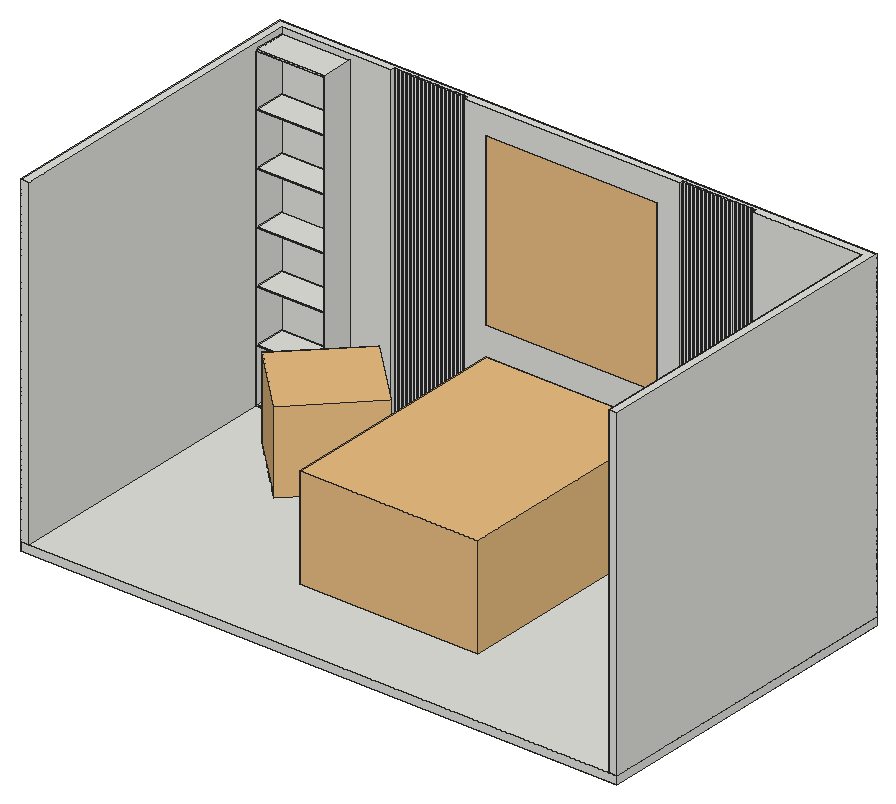
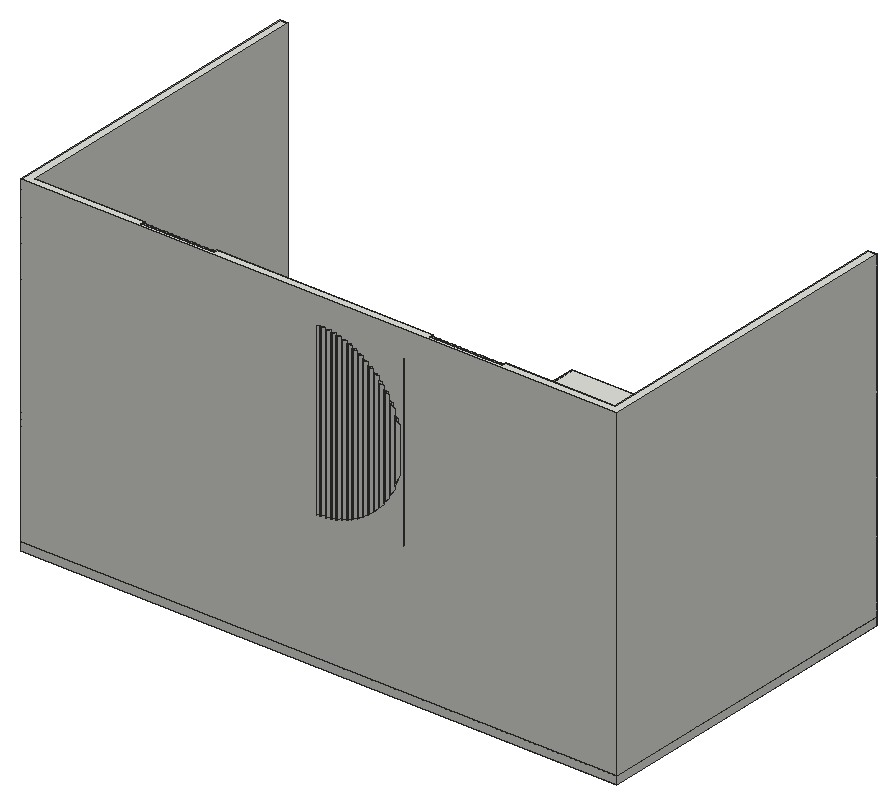
# SketchUp Ruby script. Lengths in inches.
U = 1.inch
M = Sketchup.active_model
def pt(a) = Geom::Point3d.new(a.map { |v| v * U })
def face(e, loops, mat)
  f = e.add_face(loops[0].map { |a| pt(a) })
  loops[1..].each { |l| e.add_face(l.map { |a| pt(a) }).erase! }
  f.material = f.back_material = mat if mat
  f
end
# faces: each face lists its corners as indices into pts; further lists are holes
def faces(e, pts, list, mat = nil) = list.each { |f| face(e, (f[0].is_a?(Array) ? f : [f]).map { |l| l.map { |i| pts[i] } }, mat) }
# xy, xz, yz: faces in a plane at the given z, y or x. An outline is a flat list of corners, or four numbers for a rectangle; further outlines are holes
def ring(l) = l.size == 4 ? [[l[0], l[1]], [l[2], l[1]], [l[2], l[3]], [l[0], l[3]]] : l.each_slice(2).to_a
def flat(e, list, mat, &to3) = list.each { |f| face(e, (f[0].is_a?(Array) ? f : [f]).map { |l| ring(l).map { |u, v| to3.(u, v) } }, mat) }
def xy(e, z, list, mat = nil) = flat(e, list, mat) { |x, y| [x, y, z] }
def xz(e, y, list, mat = nil) = flat(e, list, mat) { |x, z| [x, y, z] }
def yz(e, x, list, mat = nil) = flat(e, list, mat) { |y, z| [x, y, z] }
def lines(e, pts, list) = list.each { |a, b| e.add_line(pt(pts[a]), pt(pts[b])) }
# prism: a flat outline (further loops are holes) pulled along v
def prism(e, loops, v, mat = nil)
  f = face(e, loops, mat); d = Geom::Vector3d.new(v.map { |x| x * U })
  f.pushpull(f.normal.samedirection?(d) ? d.length : -d.length)
end
def box(e, o, s, mat = nil) = prism(e, [[o, [o[0] + s[0], o[1], o[2]], [o[0] + s[0], o[1] + s[1], o[2]], [o[0], o[1] + s[1], o[2]]]], [0, 0, s[2]], mat)
def at(x, y, z, deg = 0) = Geom::Transformation.translation(pt([x, y, z])) * Geom::Transformation.rotation(ORIGIN, Z_AXIS, deg.degrees)
def axes(o, x, y, z) = Geom::Transformation.new([*x, 0, *y, 0, *z, 0, *pt(o).to_a, 1])
def part(name) = M.definitions.add(name)
# library, detail: a bought-in or finely detailed component or shape, given as its bounding box
def library(name, o, s) = part(name).tap { |d| box(d.entities, o, s) }
def detail(e, o, s) = box(e.add_group.entities, o, s)
def put(e, d, t, mat = nil) = e.add_instance(d, t).tap { |i| i.material = mat if mat }
def group(e, t, mat = nil) = e.add_group.tap { |g| g.transformation = t; g.material = mat if mat }.entities
root = M.entities
M.materials.add("WALL").color = [163, 159, 147]
M.materials.add("Wood 009 27.06cm").color = [255, 255, 255]
c1 = part("Group")
box(c1.entities,[0,0,0],[440.75,240,6])
c2 = library("BED 3",[-244.73,-59.6875,196.6875],[91.01,69.4,39.64])
c3 = library("Armchair 287 004",[-17.02,-16.23,-0.09],[34.04,32.42,30.2])
c4 = part("Group25\#1")
box(c4.entities,[-26.9,-120,0],[2,240,1])
c5 = part("Group26\#1")
box(c5.entities,[-23.9,-120,0],[2,240,1])
c6 = part("Group27\#1")
box(c6.entities,[-20.9,-120,0],[2,240,1])
c7 = part("Group28\#1")
box(c7.entities,[-17.9,-120,0],[2,240,1])
c8 = part("Group29\#1")
box(c8.entities,[-14.9,-120,0],[2,240,1])
c9 = part("Group30\#1")
box(c9.entities,[-11.9,-120,0],[2,240,1])
c10 = part("Group31\#1")
box(c10.entities,[-8.9,-120,0],[2,240,1])
c11 = part("Group32\#1")
box(c11.entities,[-5.9,-120,0],[2,240,1])
c12 = part("Group33\#1")
box(c12.entities,[-2.9,-120,0],[2,240,1])
c13 = part("Group34\#1")
box(c13.entities,[0.1,-120,0],[2,240,1])
c14 = part("Group35\#1")
box(c14.entities,[3.1,-120,0],[2,240,1])
c15 = part("Group36\#1")
box(c15.entities,[6.1,-120,0],[2,240,1])
c16 = part("Group37\#1")
box(c16.entities,[9.1,-120,0],[2,240,1])
c17 = part("Group38\#1")
box(c17.entities,[12.1,-120,0],[2,240,1])
c18 = part("Group39\#1")
box(c18.entities,[15.1,-120,0],[2,240,1])
c19 = part("Group40\#1")
box(c19.entities,[18.1,-120,0],[2,240,1])
c20 = part("Group41\#1")
box(c20.entities,[21.1,-120,0],[2,240,1])
c21 = part("Group42\#1")
box(c21.entities,[24.1,-120,0],[2,240,1])
c22 = part("Group23\#1")
put(c22.entities,c4,at(0,0,0))
put(c22.entities,c5,at(0,0,0))
put(c22.entities,c6,at(0,0,0))
put(c22.entities,c7,at(0,0,0))
put(c22.entities,c8,at(0,0,0))
put(c22.entities,c9,at(0,0,0))
put(c22.entities,c10,at(0,0,0))
put(c22.entities,c11,at(0,0,0))
put(c22.entities,c12,at(0,0,0))
put(c22.entities,c13,at(0,0,0))
put(c22.entities,c14,at(0,0,0))
put(c22.entities,c15,at(0,0,0))
put(c22.entities,c16,at(0,0,0))
put(c22.entities,c17,at(0,0,0))
put(c22.entities,c18,at(0,0,0))
put(c22.entities,c19,at(0,0,0))
put(c22.entities,c20,at(0,0,0))
put(c22.entities,c21,at(0,0,0))
c23 = part("Group44\#1")
box(c23.entities,[-26.9,-120,0],[2,240,1])
c24 = part("Group45\#1")
box(c24.entities,[-23.9,-120,0],[2,240,1])
c25 = part("Group46\#1")
box(c25.entities,[-20.9,-120,0],[2,240,1])
c26 = part("Group47\#1")
box(c26.entities,[-17.9,-120,0],[2,240,1])
c27 = part("Group48\#1")
box(c27.entities,[-14.9,-120,0],[2,240,1])
c28 = part("Group49\#1")
box(c28.entities,[-11.9,-120,0],[2,240,1])
c29 = part("Group50\#1")
box(c29.entities,[-8.9,-120,0],[2,240,1])
c30 = part("Group51\#1")
box(c30.entities,[-5.9,-120,0],[2,240,1])
c31 = part("Group52\#1")
box(c31.entities,[-2.9,-120,0],[2,240,1])
c32 = part("Group53\#1")
box(c32.entities,[0.1,-120,0],[2,240,1])
c33 = part("Group54\#1")
box(c33.entities,[3.1,-120,0],[2,240,1])
c34 = part("Group55\#1")
box(c34.entities,[6.1,-120,0],[2,240,1])
c35 = part("Group56\#1")
box(c35.entities,[9.1,-120,0],[2,240,1])
c36 = part("Group57\#1")
box(c36.entities,[12.1,-120,0],[2,240,1])
c37 = part("Group58\#1")
box(c37.entities,[15.1,-120,0],[2,240,1])
c38 = part("Group59\#1")
box(c38.entities,[18.1,-120,0],[2,240,1])
c39 = part("Group60\#1")
box(c39.entities,[21.1,-120,0],[2,240,1])
c40 = part("Group61\#1")
box(c40.entities,[24.1,-120,0],[2,240,1])
c41 = part("Group42\#2")
put(c41.entities,c23,at(0,0,0))
put(c41.entities,c24,at(0,0,0))
put(c41.entities,c25,at(0,0,0))
put(c41.entities,c26,at(0,0,0))
put(c41.entities,c27,at(0,0,0))
put(c41.entities,c28,at(0,0,0))
put(c41.entities,c29,at(0,0,0))
put(c41.entities,c30,at(0,0,0))
put(c41.entities,c31,at(0,0,0))
put(c41.entities,c32,at(0,0,0))
put(c41.entities,c33,at(0,0,0))
put(c41.entities,c34,at(0,0,0))
put(c41.entities,c35,at(0,0,0))
put(c41.entities,c36,at(0,0,0))
put(c41.entities,c37,at(0,0,0))
put(c41.entities,c38,at(0,0,0))
put(c41.entities,c39,at(0,0,0))
put(c41.entities,c40,at(0,0,0))
c42 = part("Group66\#1")
p = [[0,0,0],[0,0,-7.89],[-3.85,0,-7.89],[25.04,-0.51,0],[-25.04,-0.51,0],[25.04,0.51,0],
  [25.04,0,0],[-25.04,0.51,0],[3.85,0,-7.89],[-25.04,0,0],[0,0,-12.77]]
lines(c42.entities,p,[[0,1],[1,2],[3,4],[5,6],[7,5],[1,8],[9,0],[0,6],[8,10],[4,9],[6,3],[2,10],
  [9,7]])
c43 = part("shelves")
put(c43.entities,c42,at(0,0,0))
c44 = part("Group\#5")
box(c44.entities,[0,0,0],[50.07,23.29,0.71])
c45 = library("Group\#2",[-0.5,-0.5,0],[125.9375,6,124.9375])
c46 = part("Group5\#1")
xy(c46.entities,0,[[-26.65,-23.47,-27.78,-20.53,-27.84,-20.33,-27.84,20.25,-27.32,21.79,-26.65,23.42]])
xy(c46.entities,5.875,[[-30.05,-12.08,-30.05,12.03,-30.37,10.43,-30.9,6.55,-31.19,2.63,-31.23,-1.29,-31.03,-5.21,-30.58,-9.11]])
p = [[-30.05,12.03,5.875],[-30.05,-12.08,5.875],[-29.89,-12.98,5.6],[-28.95,-16.79,3.98],[-27.78,-20.53,1.95],[-26.65,-23.47,0],
  [-26.65,23.42,0],[-27.32,21.79,1.15],[-28.57,18.07,3.33],[-29.59,14.28,5.09],[-31.03,-5.21,5.52],[-31.23,-1.29,5.875],
  [-31.19,2.63,5.8],[-30.9,6.55,5.3],[-30.37,10.43,4.375],[-29.59,14.28,3.03],[-28.57,18.07,1.27],[-27.84,20.25,0],
  [-27.84,-20.33,0],[-28.95,-16.79,1.92],[-29.89,-12.98,3.54],[-30.58,-9.11,4.74]]
faces(c46.entities,p,[[0,1,2,3,4,5,6,7,8,9],[10,11,12,13,14,15,16,17,18,19,20,21]])
c47 = part("Group6\#1")
xy(c47.entities,0,[[-22.72,-31.5,-22.89,-31.23,-23.9,-29.33,-23.9,29.35,-22.72,31.46]])
xy(c47.entities,5.875,[[-26.11,-24.78,-26.11,24.76,-27.3,21.85,-27.3,-21.79,-26.375,-24.2]])
p = [[-26.11,24.76,5.875],[-26.11,-24.78,5.875],[-24.74,-27.77,3.51],[-22.89,-31.23,0.29],[-22.72,-31.5,0],[-22.72,31.46,0],
  [-24.13,28.96,2.44],[-25.84,25.43,5.4],[-27.3,-21.79,5.875],[-27.3,21.85,5.875],[-25.84,25.43,3.35],[-24.13,28.96,0.39],
  [-23.9,29.35,0],[-23.9,-29.33,0],[-24.74,-27.77,1.45],[-26.375,-24.2,4.28]]
faces(c47.entities,p,[[0,1,2,3,4,5,6,7],[8,9,10,11,12,13,14,15]])
c48 = part("Group7\#1")
xy(c48.entities,0,[[-18.78,-37.4375,-19.97,-35.77,-19.97,35.8,-18.78,37.39]])
xy(c48.entities,5.875,[[-22.17,-32.38,-22.17,32.42,-22.2,32.38,-23.36,30.32,-23.36,-30.35,-22.89,-31.23]])
p = [[-18.78,-37.4375,0],[-18.78,37.39,0],[-20.06,35.67,2.22],[-22.17,32.42,5.875],[-22.17,-32.38,5.875],[-20.82,-34.57,3.53],
  [-23.36,-30.35,5.875],[-23.36,30.32,5.875],[-22.2,32.38,3.87],[-20.06,35.67,0.16],[-19.97,35.8,0],[-19.97,-35.77,0],
  [-20.82,-34.57,1.48],[-22.89,-31.23,5.06]]
faces(c48.entities,p,[[0,1,2,3,4,5],[6,7,8,9,10,11,12,13]])
c49 = part("Group8\#1")
xy(c49.entities,0,[[-14.84,-42.16,-16.03,-40.87,-16.03,40.82,-15.18,41.82,-14.84,42.17]])
xy(c49.entities,5.875,[[-18.23,-38.15,-18.23,38.125,-19.42,36.53,-19.42,-36.53,-18.55,-37.77]])
p = [[-14.84,-42.16,0],[-14.84,42.17,0],[-15.18,41.82,0.59],[-17.72,38.82,4.98],[-18.23,38.125,5.875],[-18.23,-38.15,5.875],
  [-16.08,-40.82,2.14],[-19.42,-36.53,5.875],[-19.42,36.53,5.875],[-17.72,38.82,2.93],[-16.03,40.82,0],[-16.03,-40.87,0],
  [-16.08,-40.82,0.08],[-18.55,-37.77,4.36]]
faces(c49.entities,p,[[0,1,2,3,4,5,6],[7,8,9,10,11,12,13]])
c50 = part("Group9\#1")
xy(c50.entities,0,[[-10.9,-46.125,-12.09,-44.98,-12.09,44.99,-10.9,46.08]])
xy(c50.entities,5.875,[[-14.3,-42.76,-14.3,42.74,-15.18,41.82,-15.48,41.46,-15.48,-41.46]])
p = [[-14.3,42.74,5.875],[-14.3,-42.76,5.875],[-13.42,-43.71,4.36],[-10.9,-46.125,0],[-10.9,46.08,0],[-12.47,44.65,2.7],
  [-15.48,-41.46,5.875],[-15.48,41.46,5.875],[-15.18,41.82,5.36],[-12.47,44.65,0.65],[-12.09,44.99,0],[-12.09,-44.98,0],
  [-13.42,-43.71,2.3]]
faces(c50.entities,p,[[0,1,2,3,4,5],[6,7,8,9,10,11,12]])
c51 = part("Group10\#1")
xy(c51.entities,0,[[-6.97,-49.43,-7.59,-48.96,-8.15,-48.49,-8.15,48.46,-6.97,49.42]])
xy(c51.entities,5.875,[[-10.36,-46.62,-10.36,46.59,-11.55,45.49,-11.55,-45.51,-10.59,-46.43]])
p = [[-6.97,-49.43,0],[-6.97,49.42,0],[-9.58,47.31,4.52],[-10.36,46.59,5.875],[-10.36,-46.62,5.875],[-7.59,-48.96,1.08],
  [-8.15,48.46,0],[-8.15,-48.49,0],[-10.59,-46.43,4.22],[-11.55,-45.51,5.875],[-11.55,45.49,5.875],[-9.58,47.31,2.46]]
faces(c51.entities,p,[[0,1,2,3,4,5],[6,7,8,9,10,11]])
c52 = part("Group11\#1")
xy(c52.entities,0,[[-3.03,-52.22,-4.22,-51.45,-4.22,51.41,-3.32,52.05,-3.03,52.23]])
xy(c52.entities,5.875,[[-6.42,-49.83,-6.42,49.85,-6.53,49.77,-7.61,48.9,-7.61,-48.95,-7.59,-48.96]])
p = [[-3.03,-52.22,0],[-3.03,52.23,0],[-3.32,52.05,0.51],[-6.42,49.85,5.875],[-6.42,-49.83,5.875],[-4.44,-51.3,2.45],
  [-4.22,51.41,0],[-4.22,-51.45,0],[-4.44,-51.3,0.39],[-7.59,-48.96,5.85],[-7.61,-48.95,5.875],[-7.61,48.9,5.875],
  [-6.53,49.77,4]]
faces(c52.entities,p,[[0,1,2,3,4,5],[6,7,8,9,10,11,12]])
c53 = part("Group12\#1")
xy(c53.entities,0,[[0.91,-54.6,-0.28,-53.93,-0.28,53.93,0.01,54.11,0.91,54.59]])
xy(c53.entities,5.875,[[-2.48,-52.57,-2.48,52.57,-3.32,52.05,-3.67,51.8,-3.67,-51.8]])
p = [[0.91,-54.6,0],[0.91,54.59,0],[0.01,54.11,1.55],[-2.48,52.57,5.875],[-2.48,-52.57,5.875],[-1.15,-53.44,3.57],
  [-3.67,-51.8,5.875],[-3.67,51.8,5.875],[-3.32,52.05,5.27],[-0.28,53.93,0],[-0.28,-53.93,0],[-1.15,-53.44,1.51]]
faces(c53.entities,p,[[0,1,2,3,4,5],[6,7,8,9,10,11]])
c54 = part("Group13\#1")
xy(c54.entities,0,[[4.85,-56.62,3.66,-56.04,3.66,56.05,4.85,56.6]])
xy(c54.entities,5.875,[[1.45,-54.91,1.45,54.89,0.27,54.25,0.27,-54.24]])
p = [[1.45,54.89,5.875],[1.45,-54.91,5.875],[2.27,-55.37,4.46],[4.85,-56.62,0],[4.85,56.6,0],[3.47,55.97,2.38],
  [3.66,56.05,0],[3.66,-56.04,0],[2.27,-55.37,2.41],[0.27,-54.24,5.875],[0.27,54.25,5.875],[3.47,55.97,0.32]]
faces(c54.entities,p,[[0,1,2,3,4,5],[6,7,8,9,10,11]])
c55 = part("Group14\#1")
xy(c55.entities,0,[[8.78,-58.3,7.6,-57.8125,7.6,57.8125,8.78,58.27]])
xy(c55.entities,5.875,[[5.39,-56.88,5.39,56.85,4.2,56.3,4.2,-56.31]])
p = [[8.78,-58.3,0],[8.78,58.27,0],[7.04,57.6,3.02],[5.39,56.85,5.875],[5.39,-56.88,5.875],[5.8,-57.08,5.16],
  [4.2,-56.31,5.875],[4.2,56.3,5.875],[7.04,57.6,0.96],[7.6,57.8125,0],[7.6,-57.8125,0],[5.8,-57.08,3.11]]
faces(c55.entities,p,[[0,1,2,3,4,5],[6,7,8,9,10,11]])
c56 = part("Group15\#1")
xy(c56.entities,0,[[12.72,-59.67,11.53,-59.27,11.53,59.27,12.72,59.64]])
xy(c56.entities,5.875,[[9.33,-58.52,9.33,58.48,8.14,58.02,8.14,-58.03]])
p = [[12.72,-59.67,0],[12.72,59.64,0],[10.71,59.01,3.49],[9.33,58.48,5.875],[9.33,-58.52,5.875],[9.43,-58.5625,5.69],
  [8.14,-58.03,5.875],[8.14,58.02,5.875],[10.71,59.01,1.43],[11.53,59.27,0],[11.53,-59.27,0],[9.43,-58.5625,3.63]]
faces(c56.entities,p,[[0,1,2,3,4,5],[6,7,8,9,10,11]])
c57 = part("Group16\#1")
xy(c57.entities,0,[[16.66,-60.76,15.47,-60.4375,15.47,60.43,16.66,60.72]])
xy(c57.entities,5.875,[[13.27,-59.85,13.27,59.81,12.08,59.4375,12.08,-59.45,13.15,-59.82]])
p = [[13.27,59.81,5.875],[13.27,-59.85,5.875],[16.66,-60.76,0],[16.66,60.72,0],[14.45,60.18,3.82],[12.08,-59.45,5.875],
  [12.08,59.4375,5.875],[14.45,60.18,1.76],[15.47,60.43,0],[15.47,-60.4375,0],[13.15,-59.82,4.01]]
faces(c57.entities,p,[[0,1,2,3,4],[5,6,7,8,9,10]])
c58 = part("Group17\#1")
xy(c58.entities,0,[[20.6,-61.57,19.41,-61.33,19.41,61.32,20.6,61.53]])
xy(c58.entities,5.875,[[17.2,-60.89,17.2,60.85,16.02,60.5625,16.02,-60.58,16.95,-60.83]])
p = [[20.6,-61.57,0],[20.6,61.53,0],[18.26,61.11,4.04],[17.2,60.85,5.875],[17.2,-60.89,5.875],[19.41,61.32,0],
  [19.41,-61.33,0],[16.95,-60.83,4.26],[16.02,-60.58,5.875],[16.02,60.5625,5.875],[18.26,61.11,1.98]]
faces(c58.entities,p,[[0,1,2,3,4],[5,6,7,8,9,10]])
c59 = part("Group18\#1")
xy(c59.entities,0,[[24.53,-62.125,23.35,-61.96,23.35,61.95,24.53,62.09]])
xy(c59.entities,5.875,[[21.14,-61.66,21.14,61.63,19.95,61.42,19.95,-61.44,20.79,-61.61]])
p = [[24.53,-62.125,0],[24.53,62.09,0],[22.13,61.81,4.16],[21.14,61.63,5.875],[21.14,-61.66,5.875],[19.95,-61.44,5.875],
  [19.95,61.42,5.875],[22.13,61.81,2.11],[23.35,61.95,0],[23.35,-61.96,0],[20.79,-61.61,4.42]]
faces(c59.entities,p,[[0,1,2,3,4],[5,6,7,8,9,10]])
c60 = part("Group19\#1")
xy(c60.entities,0,[[28.47,-62.42,27.28,-62.34,27.28,62.32,28.47,62.38]])
xy(c60.entities,5.875,[[25.08,-62.17,25.08,62.15,23.89,62.01,23.89,-62.04,24.68,-62.14]])
p = [[25.08,62.15,5.875],[25.08,-62.17,5.875],[28.47,-62.42,0],[28.47,62.38,0],[26.03,62.26,4.23],[23.89,-62.04,5.875],
  [23.89,62.01,5.875],[26.03,62.26,2.17],[27.28,62.32,0],[27.28,-62.34,0],[24.68,-62.14,4.5]]
faces(c60.entities,p,[[0,1,2,3,4],[5,6,7,8,9,10]])
c61 = part("Group20\#1")
xy(c61.entities,0,[[31.22,-62.46,31.23,62.45]])
xy(c61.entities,5.875,[[29.02,-62.4375,29.02,62.41,27.83,62.35,27.83,-62.375,28.6,-62.43]])
p = [[27.83,-62.375,5.875],[27.83,62.35,5.875],[29.95,62.46,2.2],[31.22,62.45,0],[31.22,-62.46,0],[28.6,-62.43,4.54],
  [29.02,62.41,5.875],[29.02,-62.4375,5.875],[31.23,-62.46,2.03],[31.23,62.45,2.03],[29.95,62.46,4.26]]
faces(c61.entities,p,[[0,1,2,3,4,5],[6,7,8,9,10]])
c62 = part("Group3\#1")
put(c62.entities,c46,at(0,0,0))
put(c62.entities,c47,at(0,0,0))
put(c62.entities,c48,at(0,0,0))
put(c62.entities,c49,at(0,0,0))
put(c62.entities,c50,at(0,0,0))
put(c62.entities,c51,at(0,0,0))
put(c62.entities,c52,at(0,0,0))
put(c62.entities,c53,at(0,0,0))
put(c62.entities,c54,at(0,0,0))
put(c62.entities,c55,at(0,0,0))
put(c62.entities,c56,at(0,0,0))
put(c62.entities,c57,at(0,0,0))
put(c62.entities,c58,at(0,0,0))
put(c62.entities,c59,at(0,0,0))
put(c62.entities,c60,at(0,0,0))
put(c62.entities,c61,at(0,0,0))
xy(root,0,[[0,0,0,240,440.75,240,440.75,0,434.75,0,434.75,234,353.8,234,353.8,237,299.99,237,299.99,234,140.76,234,140.76,237,86.95,237,86.95,234,6,234,6,0]])
xy(root,240,[[0,0,6,0,6,234,86.95,234,86.95,237,140.76,237,140.76,234,299.99,234,299.99,237,353.8,237,353.8,234,434.75,234,434.75,0,440.75,0,440.75,240,0,240]])
xz(root,0,[[0,0,6,240],[434.75,0,440.75,240]])
xz(root,234,[[6,0,86.95,240],[[140.76,0,299.99,240],[221.66,96.36,220.375,96.37,217.74,96.4,213.82,96.69,209.93,97.22,206.09,98,202.3,99.02,198.58,100.27,194.94,101.76,191.41,103.47,187.99,105.39,184.7,107.53,181.55,109.875,178.55,112.41,175.72,115.125,173.0625,118.02,170.59,121.07,168.32,124.27,166.25,127.61,164.4,131.06,162.77,134.63,161.36,138.3,160.1875,142.05,159.25,145.86,158.56,149.72,158.11,153.62,157.91,157.54,157.95,161.47,158.24,165.38,158.77,169.27,159.55,173.12,160.57,176.91,161.82,180.625,163.3,184.26,165.01,187.79,166.94,191.21,169.08,194.5,171.42,197.65,173.96,200.65,176.67,203.48,179.5625,206.14,182.62,208.61,185.82,210.88,189.15,212.95,192.61,214.8,196.18,216.44,199.85,217.84,203.59,219.01,207.41,219.95,211.27,220.64,215.17,221.09,219.09,221.3,220.375,221.28,223.01,221.25,226.93,220.96,230.82,220.43,234.66,219.65,238.45,218.64,242.17,217.38,245.81,215.9,249.34,214.1875,252.76,212.26,256.05,210.12,259.2,207.78,262.2,205.25,265.03,202.53,267.6875,199.64,270.16,196.59,272.43,193.39,274.5,190.05,276.35,186.59,277.98,183.02,279.39,179.36,280.5625,175.61,281.5,171.8,282.19,167.93,282.64,164.03,282.84,160.11,282.8,156.1875,282.51,152.27,281.98,148.39,281.2,144.54,280.18,140.75,278.93,137.03,277.45,133.39,275.74,129.86,273.81,126.44,271.67,123.15,269.33,120,266.79,117,264.08,114.17,261.1875,111.51,258.13,109.05,254.93,106.77,251.6,104.71,248.14,102.85,244.57,101.22,240.9,99.8125,237.16,98.64,233.34,97.71,229.48,97.01,225.58,96.5625]],[353.8,0,434.75,240]])
xz(root,239,[[221.66,96.36,225.58,96.5625,229.48,97.01,233.34,97.71,237.16,98.64,240.9,99.8125,244.57,101.22,248.14,102.85,251.6,104.71,254.93,106.77,258.13,109.05,261.1875,111.51,264.08,114.17,266.79,117,269.33,120,271.67,123.15,273.81,126.44,275.74,129.86,277.45,133.39,278.93,137.03,280.18,140.75,281.2,144.54,281.98,148.39,282.51,152.27,282.8,156.1875,282.84,160.11,282.64,164.03,282.19,167.93,281.5,171.8,280.5625,175.61,279.39,179.36,277.98,183.02,276.35,186.59,274.5,190.05,272.43,193.39,270.16,196.59,267.6875,199.64,265.03,202.53,262.2,205.25,259.2,207.78,256.05,210.12,252.76,212.26,249.34,214.1875,245.81,215.9,242.17,217.38,238.45,218.64,234.66,219.65,230.82,220.43,226.93,220.96,223.01,221.25,220.375,221.28,220.375,96.37]],"WALL")
xz(root,240,[[0,0,440.75,240]])
yz(root,0,[[0,0,240,240]])
yz(root,6,[[0,0,234,240]])
yz(root,86.95,[[234,0,237,240]])
yz(root,140.76,[[234,0,237,240]])
yz(root,299.99,[[234,0,237,240]])
yz(root,353.8,[[234,0,237,240]])
yz(root,434.75,[[0,0,234,240]])
yz(root,440.75,[[0,0,240,240]])
put(root,c1,at(0,0,-6))
put(root,c2,axes([270.05,-228.54,-371.74],[0,-1.89,0],[1.89,0,0],[0,0,1.89]))
put(root,c3,axes([83.28,178.77,0.18],[1.41421,1.41421,0],[-1.41421,1.41421,0],[0,0,2]))
put(root,c22,axes([113.85,237,120],[1,0,0],[0,0,1],[0,-1,0]),"Wood 009 27.06cm")
put(root,c41,axes([326.9,237,120],[1,0,0],[0,0,1],[0,-1,0]),"Wood 009 27.06cm")
g1 = group(root,at(6,210.41,0))
xy(g1,0,[[0,0,50.62,23.59]])
xy(g1,0.7,[[0.7,0,49.92,22.9]])
xy(g1,235.25,[[0.7,0,49.92,22.9]])
xy(g1,235.94,[[0,0,50.62,23.59]])
xz(g1,0,[[[0,0,50.62,235.94],[0.7,0.7,49.92,235.25]]])
xz(g1,22.9,[[0.7,0.7,49.92,235.25]])
xz(g1,23.59,[[0,0,50.62,235.94]])
yz(g1,0,[[0,0,23.59,235.94]])
yz(g1,0.7,[[0,0.7,22.9,235.25]])
yz(g1,49.92,[[0,0.7,22.9,235.25]])
yz(g1,50.62,[[0,0,23.59,235.94]])
put(root,c43,axes([31.3125,232.8,36.54],[0.9831,0,0],[0,-0.9831,0],[0,0,0.9831]))
put(root,c44,axes([6.7,210.41,39.49],[0.9831,0,0],[0,0.9831,0],[0,0,0.9831]))
put(root,c43,axes([31.3125,232.8,75.61],[0.9831,0,0],[0,-0.9831,0],[0,0,0.9831]))
put(root,c44,axes([6.7,210.41,78.57],[0.9831,0,0],[0,0.9831,0],[0,0,0.9831]))
put(root,c45,at(157.91,234,96.36))
put(root,c62,axes([189.14,241.9375,158.83],[1,0,0],[0,0,1],[0,-1,0]))
put(root,c43,axes([31.3125,232.8,113.59],[0.9831,0,0],[0,-0.9831,0],[0,0,0.9831]))
g2 = group(root,at(6.7,210.41,117.65))
box(g2,[0,0,0],[49.23,22.9,0.7])
put(root,c43,axes([31.3125,232.8,155.24],[0.9831,0,0],[0,-0.9831,0],[0,0,0.9831]))
put(root,c44,axes([6.7,210.41,156.73],[0.9831,0,0],[0,0.9831,0],[0,0,0.9831]))
put(root,c43,axes([31.3125,232.8,195.31],[0.9831,0,0],[0,-0.9831,0],[0,0,0.9831]))
put(root,c44,axes([6.7,210.41,195.81],[0.9831,0,0],[0,0.9831,0],[0,0,0.9831]))
put(root,c43,axes([31.3125,232.8,234.75],[0.9831,0,0],[0,-0.9831,0],[0,0,0.9831]))
